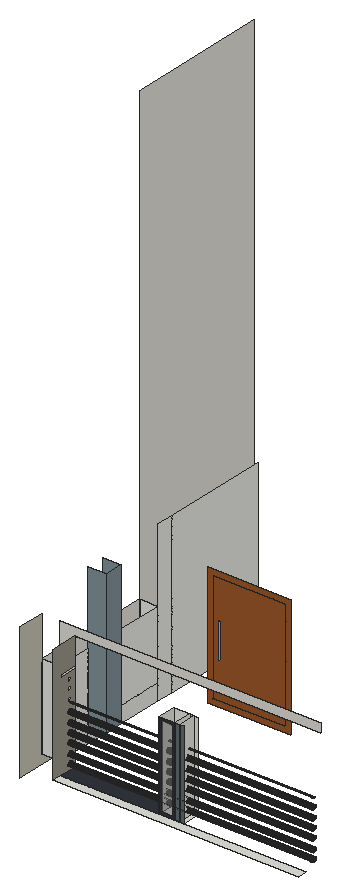
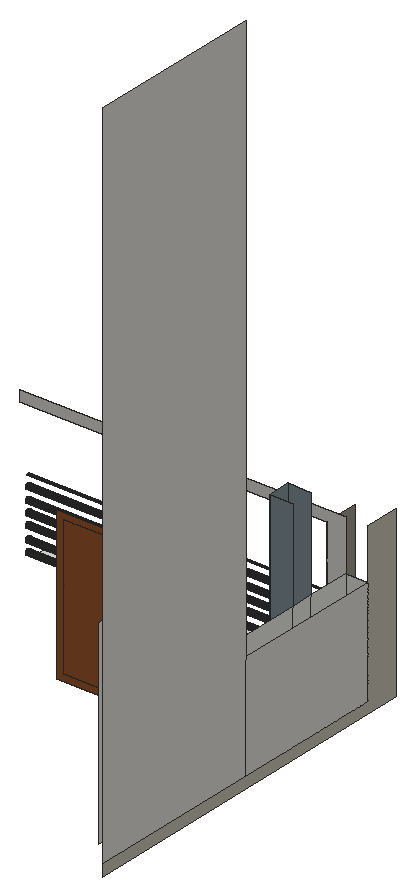
# SketchUp Ruby script. Lengths in inches.
U = 1.inch
M = Sketchup.active_model
def pt(a) = Geom::Point3d.new(a.map { |v| v * U })
def face(e, loops, mat)
  f = e.add_face(loops[0].map { |a| pt(a) })
  loops[1..].each { |l| e.add_face(l.map { |a| pt(a) }).erase! }
  f.material = f.back_material = mat if mat
  f
end
# faces: each face lists its corners as indices into pts; further lists are holes
def faces(e, pts, list, mat = nil) = list.each { |f| face(e, (f[0].is_a?(Array) ? f : [f]).map { |l| l.map { |i| pts[i] } }, mat) }
# xy, xz, yz: faces in a plane at the given z, y or x. An outline is a flat list of corners, or four numbers for a rectangle; further outlines are holes
def ring(l) = l.size == 4 ? [[l[0], l[1]], [l[2], l[1]], [l[2], l[3]], [l[0], l[3]]] : l.each_slice(2).to_a
def flat(e, list, mat, &to3) = list.each { |f| face(e, (f[0].is_a?(Array) ? f : [f]).map { |l| ring(l).map { |u, v| to3.(u, v) } }, mat) }
def xy(e, z, list, mat = nil) = flat(e, list, mat) { |x, y| [x, y, z] }
def xz(e, y, list, mat = nil) = flat(e, list, mat) { |x, z| [x, y, z] }
def yz(e, x, list, mat = nil) = flat(e, list, mat) { |y, z| [x, y, z] }
def lines(e, pts, list) = list.each { |a, b| e.add_line(pt(pts[a]), pt(pts[b])) }
# prism: a flat outline (further loops are holes) pulled along v
def prism(e, loops, v, mat = nil)
  f = face(e, loops, mat); d = Geom::Vector3d.new(v.map { |x| x * U })
  f.pushpull(f.normal.samedirection?(d) ? d.length : -d.length)
end
def box(e, o, s, mat = nil) = prism(e, [[o, [o[0] + s[0], o[1], o[2]], [o[0] + s[0], o[1] + s[1], o[2]], [o[0], o[1] + s[1], o[2]]]], [0, 0, s[2]], mat)
def at(x, y, z, deg = 0) = Geom::Transformation.translation(pt([x, y, z])) * Geom::Transformation.rotation(ORIGIN, Z_AXIS, deg.degrees)
def axes(o, x, y, z) = Geom::Transformation.new([*x, 0, *y, 0, *z, 0, *pt(o).to_a, 1])
def part(name) = M.definitions.add(name)
# library, detail: a bought-in or finely detailed component or shape, given as its bounding box
def library(name, o, s) = part(name).tap { |d| box(d.entities, o, s) }
def detail(e, o, s) = box(e.add_group.entities, o, s)
def put(e, d, t, mat = nil) = e.add_instance(d, t).tap { |i| i.material = mat if mat }
def group(e, t, mat = nil) = e.add_group.tap { |g| g.transformation = t; g.material = mat if mat }.entities
root = M.entities
M.materials.add("[Formica Graystone]").color = [193, 189, 175]
M.materials.add("[Formica Graystone]1").color = [149, 146, 135]
M.materials.add("[Formica Laminate Dark]").color = [50, 53, 60]
M.materials.add("[Formica Speckled Grey]").color = [127, 142, 150]
M.materials.add("[Formica Speckled Grey]1").color = [94, 105, 111]
M.materials.add("[Terrazzo Tile Light]").color = [219, 217, 210]
M.materials.add("[Translucent Glass Gray]").color = [128, 128, 128]
M.materials["[Translucent Glass Gray]"].alpha = 0.5
M.materials.add("[Wood Cherry Original]").color = [152, 86, 42]
M.materials.add("[Wood Floor Light]").color = [204, 176, 127]
xy(root,9,[[32.82,13.1875,277.85,22.75],[131.17,22.75,146.95,40.6875],[146.95,22.75,151.42,40.6875],[151.42,22.75,155.89,40.6875],[0,40.6875,17.9375,162.27]])
xy(root,9,[[32.82,22.75,131.17,40.6875]],"[Formica Laminate Dark]")
xy(root,25.4375,[[17.9375,75.25,36.375,93.6875]])
xz(root,22.75,[[[131.17,9,146.95,96.38],[133.64,11.46,144.49,93.92]]],"[Formica Laminate Dark]")
xz(root,22.75,[[146.95,9,151.42,96.38],[151.42,9,155.89,96.38]],"[Formica Speckled Grey]1")
xz(root,22.75,[[133.64,11.46,144.49,93.92]],"[Translucent Glass Gray]")
xz(root,40.6875,[[0,9,17.9375,93.9375],[131.17,9,146.95,96.38],[146.95,9,151.42,96.38],[151.42,9,155.89,96.38]])
xz(root,40.6875,[[17.9375,9,17.9375,134.5,277.85,134.5,277.85,125.79,32.82,125.79,32.82,9]],"[Terrazzo Tile Light]")
xz(root,75.25,[[17.9375,25.4375,36.375,167.375]],"[Formica Speckled Grey]")
xz(root,93.6875,[[17.9375,25.4375,36.375,167.375]],"[Formica Speckled Grey]")
xz(root,162.27,[[0,9,17.9375,93.9375]])
xz(root,162.27,[[[67.875,25.4375,151.125,146.5],[73.24,30.81,145.75,141.13]],[[73.24,30.81,145.75,141.13],[77.73,66.83,81.36,103.21]]],"[Wood Cherry Original]")
xz(root,162.27,[[77.73,66.83,81.36,103.21]],"[Wood Floor Light]")
yz(root,0,[[13.1875,0,13.1875,134.5,40.6875,134.5,40.6875,9,305.18,9,305.18,0]],"[Formica Graystone]")
yz(root,0,[[40.6875,9,162.27,93.9375],[162.27,9,305.18,549.4375]],"[Terrazzo Tile Light]")
yz(root,17.9375,[[40.6875,9,75.25,93.9375],[75.25,9,162.27,25.4375],[162.27,9,180.28,167.375],[180.28,9,287.24,167.375],[75.25,25.4375,93.6875,93.9375],
  [93.6875,25.4375,162.27,93.9375]])
yz(root,32.82,[[[13.1875,9,40.6875,9,40.6875,96.38,22.75,96.38,22.75,99.34,40.6875,99.34,40.6875,125.79,13.1875,125.79],[33.12,88.66,32.57,88.74,32.05,88.95,31.61,89.29,31.28,89.73,31.06,90.24,30.99,90.79,31.06,91.34,31.28,91.85,31.61,92.29,32.05,92.63,32.57,92.84,33.12,92.91,33.67,92.84,34.18,92.63,34.62,92.29,34.96,91.85,35.17,91.34,35.24,90.79,35.17,90.24,34.96,89.73,34.62,89.29,34.18,88.95,33.67,88.74],[33.12,80.16,32.57,80.24,32.05,80.45,31.61,80.79,31.28,81.23,31.06,81.74,30.99,82.29,31.06,82.84,31.28,83.35,31.61,83.79,32.05,84.13,32.57,84.34,33.12,84.41,33.67,84.34,34.18,84.13,34.62,83.79,34.96,83.35,35.17,82.84,35.24,82.29,35.17,81.74,34.96,81.23,34.62,80.79,34.18,80.45,33.67,80.24],[33.12,70.48,32.57,70.55,32.05,70.76,31.61,71.1,31.28,71.54,31.06,72.05,30.99,72.6,31.06,73.15,31.28,73.66,31.61,74.1,32.05,74.44,32.57,74.65,33.12,74.73,33.67,74.65,34.18,74.44,34.62,74.1,34.96,73.66,35.17,73.15,35.24,72.6,35.17,72.05,34.96,71.54,34.62,71.1,34.18,70.76,33.67,70.55],[33.12,60.04,32.57,60.11,32.05,60.32,31.61,60.66,31.28,61.1,31.06,61.61,30.99,62.16,31.06,62.71,31.28,63.23,31.61,63.67,32.05,64,32.57,64.22,33.12,64.29,33.67,64.22,34.18,64,34.62,63.67,34.96,63.23,35.17,62.71,35.24,62.16,35.17,61.61,34.96,61.1,34.62,60.66,34.18,60.32,33.67,60.11],[33.12,32.23,32.57,32.3,32.05,32.51,31.61,32.85,31.28,33.29,31.06,33.8,30.99,34.35,31.06,34.9,31.28,35.41,31.61,35.85,32.05,36.19,32.57,36.4,33.12,36.48,33.67,36.4,34.18,36.19,34.62,35.85,34.96,35.41,35.17,34.9,35.24,34.35,35.17,33.8,34.96,33.29,34.62,32.85,34.18,32.51,33.67,32.3],[33.12,13.1,32.57,13.17,32.05,13.39,31.61,13.72,31.28,14.16,31.06,14.68,30.99,15.23,31.06,15.78,31.28,16.29,31.61,16.73,32.05,17.07,32.57,17.28,33.12,17.35,33.67,17.28,34.18,17.07,34.62,16.73,34.96,16.29,35.17,15.78,35.24,15.23,35.17,14.68,34.96,14.16,34.62,13.72,34.18,13.39,33.67,13.17],[33.12,21.91,32.57,21.99,32.05,22.2,31.61,22.54,31.28,22.98,31.06,23.49,30.99,24.04,31.06,24.59,31.28,25.1,31.61,25.54,32.05,25.88,32.57,26.09,33.12,26.16,33.67,26.09,34.18,25.88,34.62,25.54,34.96,25.1,35.17,24.59,35.24,24.04,35.17,23.49,34.96,22.98,34.62,22.54,34.18,22.2,33.67,21.99],[33.12,50.23,32.57,50.3,32.05,50.51,31.61,50.85,31.28,51.29,31.06,51.8,30.99,52.35,31.06,52.9,31.28,53.41,31.61,53.85,32.05,54.19,32.57,54.4,33.12,54.48,33.67,54.4,34.18,54.19,34.62,53.85,34.96,53.41,35.17,52.9,35.24,52.35,35.17,51.8,34.96,51.29,34.62,50.85,34.18,50.51,33.67,50.3],[33.12,41.23,32.57,41.3,32.05,41.51,31.61,41.85,31.28,42.29,31.06,42.8,30.99,43.35,31.06,43.9,31.28,44.41,31.61,44.85,32.05,45.19,32.57,45.4,33.12,45.48,33.67,45.4,34.18,45.19,34.62,44.85,34.96,44.41,35.17,43.9,35.24,43.35,35.17,42.8,34.96,42.29,34.62,41.85,34.18,41.51,33.67,41.3]]],"[Formica Graystone]1")
yz(root,36.375,[[75.25,25.4375,93.6875,167.375]],"[Formica Speckled Grey]")
yz(root,131.17,[[22.75,9,40.6875,96.38]])
yz(root,146.95,[[22.75,9,40.6875,96.38]])
yz(root,151.42,[[22.75,9,40.6875,96.38]])
p = [[277.85,33.12,13.1],[277.85,32.57,13.17],[32.82,32.57,13.17],[32.82,33.12,13.1],[277.85,33.67,13.17],[32.82,33.67,13.17],
  [277.85,32.05,13.39],[32.82,32.05,13.39],[277.85,34.18,13.39],[32.82,34.18,13.39],[277.85,31.61,13.72],[32.82,31.61,13.72],
  [277.85,34.62,13.72],[32.82,34.62,13.72],[277.85,31.28,14.16],[32.82,31.28,14.16],[277.85,34.96,14.16],[32.82,34.96,14.16],
  [277.85,31.06,14.68],[32.82,31.06,14.68],[277.85,35.17,14.68],[32.82,35.17,14.68],[277.85,30.99,15.23],[32.82,30.99,15.23],
  [277.85,35.24,15.23],[32.82,35.24,15.23],[277.85,31.06,15.78],[32.82,31.06,15.78],[277.85,35.17,15.78],[32.82,35.17,15.78],
  [277.85,31.28,16.29],[32.82,31.28,16.29],[277.85,34.96,16.29],[32.82,34.96,16.29],[277.85,31.61,16.73],[32.82,31.61,16.73],
  [277.85,34.62,16.73],[32.82,34.62,16.73],[277.85,32.05,17.07],[32.82,32.05,17.07],[277.85,34.18,17.07],[32.82,34.18,17.07],
  [277.85,32.57,17.28],[32.82,32.57,17.28],[277.85,33.67,17.28],[32.82,33.67,17.28],[277.85,33.12,17.35],[32.82,33.12,17.35],
  [277.85,33.12,21.91],[277.85,32.57,21.99],[32.82,32.57,21.99],[32.82,33.12,21.91],[277.85,33.67,21.99],[32.82,33.67,21.99],
  [277.85,32.05,22.2],[32.82,32.05,22.2],[277.85,34.18,22.2],[32.82,34.18,22.2],[277.85,31.61,22.54],[32.82,31.61,22.54],
  [277.85,34.62,22.54],[32.82,34.62,22.54],[277.85,31.28,22.98],[32.82,31.28,22.98],[277.85,34.96,22.98],[32.82,34.96,22.98],
  [277.85,31.06,23.49],[32.82,31.06,23.49],[277.85,35.17,23.49],[32.82,35.17,23.49],[277.85,30.99,24.04],[32.82,30.99,24.04],
  [277.85,35.24,24.04],[32.82,35.24,24.04],[277.85,31.06,24.59],[32.82,31.06,24.59],[277.85,35.17,24.59],[32.82,35.17,24.59],
  [277.85,31.28,25.1],[32.82,31.28,25.1],[277.85,34.96,25.1],[32.82,34.96,25.1],[277.85,31.61,25.54],[32.82,31.61,25.54],
  [277.85,34.62,25.54],[32.82,34.62,25.54],[277.85,32.05,25.88],[32.82,32.05,25.88],[277.85,34.18,25.88],[32.82,34.18,25.88],
  [277.85,32.57,26.09],[32.82,32.57,26.09],[277.85,33.67,26.09],[32.82,33.67,26.09],[277.85,33.12,26.16],[32.82,33.12,26.16],
  [277.85,33.12,32.23],[277.85,32.57,32.3],[32.82,32.57,32.3],[32.82,33.12,32.23],[277.85,33.67,32.3],[32.82,33.67,32.3],
  [277.85,32.05,32.51],[32.82,32.05,32.51],[277.85,34.18,32.51],[32.82,34.18,32.51],[277.85,31.61,32.85],[32.82,31.61,32.85],
  [277.85,34.62,32.85],[32.82,34.62,32.85],[277.85,31.28,33.29],[32.82,31.28,33.29],[277.85,34.96,33.29],[32.82,34.96,33.29],
  [277.85,31.06,33.8],[32.82,31.06,33.8],[277.85,35.17,33.8],[32.82,35.17,33.8],[277.85,30.99,34.35],[32.82,30.99,34.35],
  [277.85,35.24,34.35],[32.82,35.24,34.35],[277.85,31.06,34.9],[32.82,31.06,34.9],[277.85,35.17,34.9],[32.82,35.17,34.9],
  [277.85,31.28,35.41],[32.82,31.28,35.41],[277.85,34.96,35.41],[32.82,34.96,35.41],[277.85,31.61,35.85],[32.82,31.61,35.85],
  [277.85,34.62,35.85],[32.82,34.62,35.85],[277.85,32.05,36.19],[32.82,32.05,36.19],[277.85,34.18,36.19],[32.82,34.18,36.19],
  [277.85,32.57,36.4],[32.82,32.57,36.4],[277.85,33.67,36.4],[32.82,33.67,36.4],[277.85,33.12,36.48],[32.82,33.12,36.48],
  [277.85,33.12,41.23],[277.85,32.57,41.3],[32.82,32.57,41.3],[32.82,33.12,41.23],[277.85,33.67,41.3],[32.82,33.67,41.3],
  [277.85,32.05,41.51],[32.82,32.05,41.51],[277.85,34.18,41.51],[32.82,34.18,41.51],[277.85,31.61,41.85],[32.82,31.61,41.85],
  [277.85,34.62,41.85],[32.82,34.62,41.85],[277.85,31.28,42.29],[32.82,31.28,42.29],[277.85,34.96,42.29],[32.82,34.96,42.29],
  [277.85,31.06,42.8],[32.82,31.06,42.8],[277.85,35.17,42.8],[32.82,35.17,42.8],[277.85,30.99,43.35],[32.82,30.99,43.35],
  [277.85,35.24,43.35],[32.82,35.24,43.35],[277.85,31.06,43.9],[32.82,31.06,43.9],[277.85,35.17,43.9],[32.82,35.17,43.9],
  [277.85,31.28,44.41],[32.82,31.28,44.41],[277.85,34.96,44.41],[32.82,34.96,44.41],[277.85,31.61,44.85],[32.82,31.61,44.85],
  [277.85,34.62,44.85],[32.82,34.62,44.85],[277.85,32.05,45.19],[32.82,32.05,45.19],[277.85,34.18,45.19],[32.82,34.18,45.19],
  [277.85,32.57,45.4],[32.82,32.57,45.4],[277.85,33.67,45.4],[32.82,33.67,45.4],[277.85,33.12,45.48],[32.82,33.12,45.48],
  [277.85,33.12,50.23],[277.85,32.57,50.3],[32.82,32.57,50.3],[32.82,33.12,50.23],[277.85,33.67,50.3],[32.82,33.67,50.3],
  [277.85,32.05,50.51],[32.82,32.05,50.51],[277.85,34.18,50.51],[32.82,34.18,50.51],[277.85,31.61,50.85],[32.82,31.61,50.85],
  [277.85,34.62,50.85],[32.82,34.62,50.85],[277.85,31.28,51.29],[32.82,31.28,51.29],[277.85,34.96,51.29],[32.82,34.96,51.29],
  [277.85,31.06,51.8],[32.82,31.06,51.8],[277.85,35.17,51.8],[32.82,35.17,51.8],[277.85,30.99,52.35],[32.82,30.99,52.35],
  [277.85,35.24,52.35],[32.82,35.24,52.35],[277.85,31.06,52.9],[32.82,31.06,52.9],[277.85,35.17,52.9],[32.82,35.17,52.9],
  [277.85,31.28,53.41],[32.82,31.28,53.41],[277.85,34.96,53.41],[32.82,34.96,53.41],[277.85,31.61,53.85],[32.82,31.61,53.85],
  [277.85,34.62,53.85],[32.82,34.62,53.85],[277.85,32.05,54.19],[32.82,32.05,54.19],[277.85,34.18,54.19],[32.82,34.18,54.19],
  [277.85,32.57,54.4],[32.82,32.57,54.4],[277.85,33.67,54.4],[32.82,33.67,54.4],[277.85,33.12,54.48],[32.82,33.12,54.48],
  [277.85,33.12,60.04],[277.85,32.57,60.11],[32.82,32.57,60.11],[32.82,33.12,60.04],[277.85,33.67,60.11],[32.82,33.67,60.11],
  [277.85,32.05,60.32],[32.82,32.05,60.32],[277.85,34.18,60.32],[32.82,34.18,60.32],[277.85,31.61,60.66],[32.82,31.61,60.66],
  [277.85,34.62,60.66],[32.82,34.62,60.66],[277.85,31.28,61.1],[32.82,31.28,61.1],[277.85,34.96,61.1],[32.82,34.96,61.1],
  [277.85,31.06,61.61],[32.82,31.06,61.61],[277.85,35.17,61.61],[32.82,35.17,61.61],[277.85,30.99,62.16],[32.82,30.99,62.16],
  [277.85,35.24,62.16],[32.82,35.24,62.16],[277.85,31.06,62.71],[32.82,31.06,62.71],[277.85,35.17,62.71],[32.82,35.17,62.71],
  [277.85,31.28,63.23],[32.82,31.28,63.23],[277.85,34.96,63.23],[32.82,34.96,63.23],[277.85,31.61,63.67],[32.82,31.61,63.67],
  [277.85,34.62,63.67],[32.82,34.62,63.67],[277.85,32.05,64],[32.82,32.05,64],[277.85,34.18,64],[32.82,34.18,64],
  [277.85,32.57,64.22],[32.82,32.57,64.22],[277.85,33.67,64.22],[32.82,33.67,64.22],[277.85,33.12,64.29],[32.82,33.12,64.29],
  [277.85,32.57,70.55],[277.85,32.05,70.76],[32.82,32.05,70.76],[32.82,32.57,70.55],[277.85,33.12,70.48],[32.82,33.12,70.48],
  [277.85,33.67,70.55],[32.82,33.67,70.55],[277.85,34.18,70.76],[32.82,34.18,70.76]]
faces(root,p,[[0,1,2,3],[4,0,3,5],[1,6,7,2],[8,4,5,9],[6,10,11,7],[12,8,9,13],[10,14,15,11],[16,12,13,17],
  [14,18,19,15],[20,16,17,21],[18,22,23,19],[24,20,21,25],[22,26,27,23],[28,24,25,29],[26,30,31,27],[32,28,29,33],
  [30,34,35,31],[36,32,33,37],[34,38,39,35],[40,36,37,41],[38,42,43,39],[44,40,41,45],[42,46,47,43],[46,44,45,47],
  [48,49,50,51],[52,48,51,53],[49,54,55,50],[56,52,53,57],[54,58,59,55],[60,56,57,61],[58,62,63,59],[64,60,61,65],
  [62,66,67,63],[68,64,65,69],[66,70,71,67],[72,68,69,73],[70,74,75,71],[76,72,73,77],[74,78,79,75],[80,76,77,81],
  [78,82,83,79],[84,80,81,85],[82,86,87,83],[88,84,85,89],[86,90,91,87],[92,88,89,93],[90,94,95,91],[94,92,93,95],
  [96,97,98,99],[100,96,99,101],[97,102,103,98],[104,100,101,105],[102,106,107,103],[108,104,105,109],[106,110,111,107],[112,108,109,113],
  [110,114,115,111],[116,112,113,117],[114,118,119,115],[120,116,117,121],[118,122,123,119],[124,120,121,125],[122,126,127,123],[128,124,125,129],
  [126,130,131,127],[132,128,129,133],[130,134,135,131],[136,132,133,137],[134,138,139,135],[140,136,137,141],[138,142,143,139],[142,140,141,143],
  [144,145,146,147],[148,144,147,149],[145,150,151,146],[152,148,149,153],[150,154,155,151],[156,152,153,157],[154,158,159,155],[160,156,157,161],
  [158,162,163,159],[164,160,161,165],[162,166,167,163],[168,164,165,169],[166,170,171,167],[172,168,169,173],[170,174,175,171],[176,172,173,177],
  [174,178,179,175],[180,176,177,181],[178,182,183,179],[184,180,181,185],[182,186,187,183],[188,184,185,189],[186,190,191,187],[190,188,189,191],
  [192,193,194,195],[196,192,195,197],[193,198,199,194],[200,196,197,201],[198,202,203,199],[204,200,201,205],[202,206,207,203],[208,204,205,209],
  [206,210,211,207],[212,208,209,213],[210,214,215,211],[216,212,213,217],[214,218,219,215],[220,216,217,221],[218,222,223,219],[224,220,221,225],
  [222,226,227,223],[228,224,225,229],[226,230,231,227],[232,228,229,233],[230,234,235,231],[236,232,233,237],[234,238,239,235],[238,236,237,239],
  [240,241,242,243],[244,240,243,245],[241,246,247,242],[248,244,245,249],[246,250,251,247],[252,248,249,253],[250,254,255,251],[256,252,253,257],
  [254,258,259,255],[260,256,257,261],[258,262,263,259],[264,260,261,265],[262,266,267,263],[268,264,265,269],[266,270,271,267],[272,268,269,273],
  [270,274,275,271],[276,272,273,277],[274,278,279,275],[280,276,277,281],[278,282,283,279],[284,280,281,285],[282,286,287,283],[286,284,285,287],
  [288,289,290,291],[292,288,291,293],[294,292,293,295],[296,294,295,297]],"[Formica Laminate Dark]")
